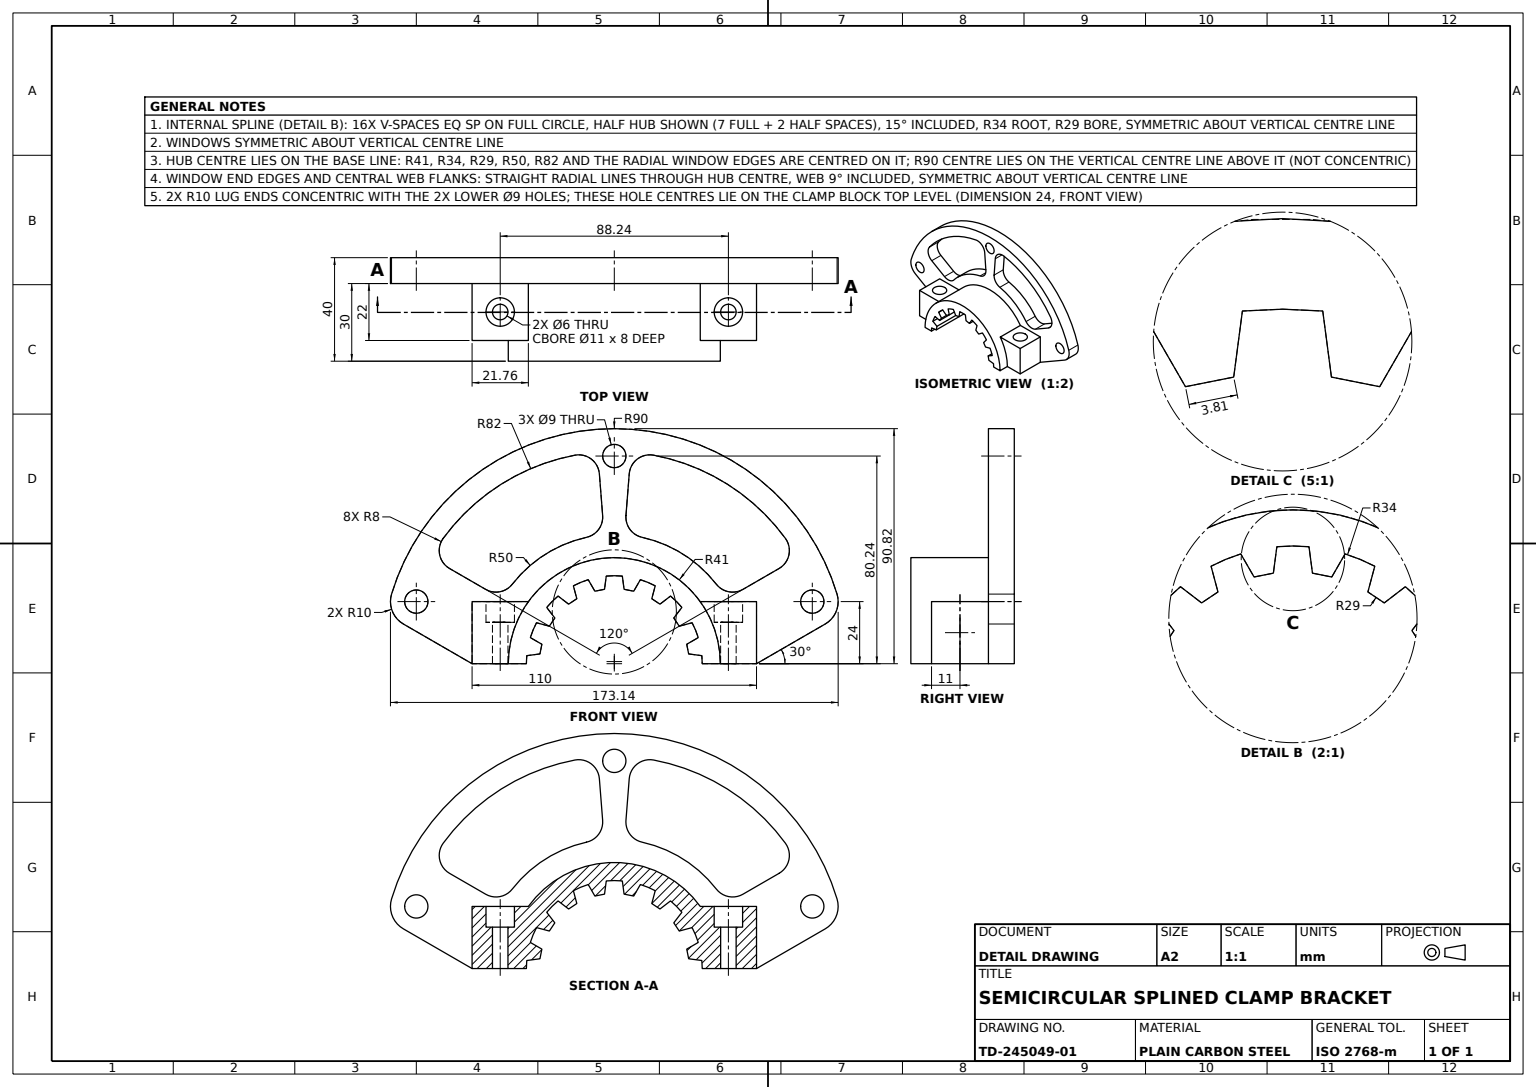
solid
v1 (-10.76075,48.828334,10)
v2 (-10.76075,48.828334,0)
e1 v1 v2 LINE
v3 (-39.439114,30.733635,0)
e2 v3 v2 CIRCLE(AX(P(0,0,0),D(0,0,-1),D(-1,0,0)),50)
v4 (-39.439114,30.733635,10)
e3 v4 v3 LINE
e4 v4 v1 CIRCLE(AX(P(0,0,10),D(0,0,-1),D(-1,0,0)),50)
face CYL(AX(P(0,0,10),D(0,0,-1),D(-1,0,0)),50) [e1 -e2 -e3 e4]
v5 (44.12077,16,26.5)
v6 (44.12077,24,26.5)
e5 v5 v6 LINE
v7 (44.12077,16,15.5)
e6 v7 v5 CIRCLE(AX(P(44.12077,16,21),D(0,1,0),D(0,0,1)),5.5)
v8 (44.12077,24,15.5)
e7 v7 v8 LINE
e8 v8 v6 CIRCLE(AX(P(44.12077,24,21),D(0,1,0),D(0,0,1)),5.5)
face CYL(AX(P(44.12077,24,21),D(0,1,0),D(0,0,1)),5.5) rev [-e5 -e6 e7 e8]
v9 (28.010307,7.511504,40)
v10 (28.752678,3.779355,40)
e9 v9 v10 CIRCLE(AX(P(0,0,40),D(0,0,-1),D(1,0,0)),29)
v11 (28.010307,7.511504,0)
e10 v11 v9 LINE
v12 (28.752678,3.779355,0)
e11 v11 v12 CIRCLE(AX(P(0,0,0),D(0,0,-1),D(1,0,0)),29)
e12 v12 v10 LINE
face CYL(AX(P(0,0,0),D(0,0,1),D(1,0,0)),29) rev [-e9 -e10 e11 e12]
v13 (-86.140372,26.897075,10)
v14 (-86.140372,26.897075,0)
e13 v13 v14 LINE
v15 (-86.569219,24,0)
e14 v14 v15 CIRCLE(AX(P(-76.569219,24,0),D(0,0,1),D(-1,0,0)),10)
v16 (-86.569219,24,10)
e15 v16 v15 LINE
e16 v13 v16 CIRCLE(AX(P(-76.569219,24,10),D(0,0,1),D(-1,0,0)),10)
face CYL(AX(P(-76.569219,24,10),D(0,0,-1),D(-1,0,0)),10) [e13 e14 -e15 -e16]
v17 (-33.24154,24,10)
v18 (-33.24154,24,32)
e17 v17 v18 LINE
v19 (-41,0,32)
e18 v18 v19 CIRCLE(AX(P(0,0,32),D(0,0,1),D(-1,0,0)),41)
v20 (-41,0,40)
e19 v20 v19 LINE
v21 (41,0,40)
e20 v21 v20 CIRCLE(AX(P(0,0,40),D(0,0,1),D(-1,0,0)),41)
v22 (41,0,32)
e21 v21 v22 LINE
v23 (33.24154,24,32)
e22 v22 v23 CIRCLE(AX(P(0,0,32),D(0,0,1),D(-1,0,0)),41)
v24 (33.24154,24,10)
e23 v23 v24 LINE
e24 v24 v17 CIRCLE(AX(P(0,0,10),D(0,0,1),D(-1,0,0)),41)
face CYL(AX(P(0,0,40),D(0,0,-1),D(-1,0,0)),41) [e17 e18 -e19 -e20 e21 e22 e23 e24]
v25 (-81.569219,15.339746,0)
e25 v15 v25 CIRCLE(AX(P(-76.569219,24,0),D(0,0,1),D(-1,0,0)),10)
v26 (-81.569219,15.339746,10)
e26 v26 v25 LINE
e27 v16 v26 CIRCLE(AX(P(-76.569219,24,10),D(0,0,1),D(-1,0,0)),10)
face CYL(AX(P(-76.569219,24,10),D(0,0,-1),D(-1,0,0)),10) [e15 e25 -e26 -e27]
v27 (32.469549,10.086049,0)
v28 (32.469549,10.086049,40)
e28 v27 v28 LINE
v29 (30.091352,15.827525,40)
e29 v29 v28 CIRCLE(AX(P(0,0,40),D(0,0,-1),D(1,0,0)),34)
v30 (30.091352,15.827525,0)
e30 v30 v29 LINE
e31 v30 v27 CIRCLE(AX(P(0,0,0),D(0,0,-1),D(1,0,0)),34)
face CYL(AX(P(0,0,0),D(0,0,1),D(1,0,0)),34) rev [e28 -e29 -e30 e31]
v31 (10.76075,48.828334,0)
v32 (39.439114,30.733635,0)
e32 v31 v32 CIRCLE(AX(P(0,0,0),D(0,0,-1),D(-1,0,0)),50)
v33 (10.76075,48.828334,10)
e33 v33 v31 LINE
v34 (39.439114,30.733635,10)
e34 v33 v34 CIRCLE(AX(P(0,0,10),D(0,0,-1),D(-1,0,0)),50)
e35 v34 v32 LINE
face CYL(AX(P(0,0,10),D(0,0,-1),D(-1,0,0)),50) [-e32 -e33 e34 e35]
v35 (-55,0,0)
e36 v25 v35 LINE
v36 (-55,0,10)
e37 v36 v35 LINE
e38 v26 v36 LINE
face PLANE(AX(P(-55,0,10),D(0.5,0.866025404,0),D(-0.866025404,0.5,0))) rev [e26 e36 -e37 -e38]
v37 (-25.117714,14.494842,0)
v38 (-25.117714,14.494842,40)
e39 v37 v38 LINE
v39 (-30.091352,15.827525,40)
e40 v39 v38 LINE
v40 (-30.091352,15.827525,0)
e41 v40 v39 LINE
e42 v40 v37 LINE
face PLANE(AX(P(1.941143,7.244444,0),D(-0.258819045,-0.965925826,0),D(0.965925826,-0.258819045,0))) [e39 -e40 -e41 e42]
v41 (3.107264,33.857716,40)
v42 (3.779355,28.752678,40)
e43 v41 v42 LINE
v43 (3.107264,33.857716,0)
e44 v43 v41 LINE
v44 (3.779355,28.752678,0)
e45 v43 v44 LINE
e46 v44 v42 LINE
face PLANE(AX(P(7.435836,0.978946,0),D(-0.991444861,-0.130526192,0),D(0.130526192,-0.991444861,0))) [-e43 -e44 e45 e46]
v45 (17.658806,23.003621,0)
v46 (17.658806,23.003621,40)
e47 v45 v46 LINE
v47 (14.494842,25.117714,40)
e48 v47 v46 CIRCLE(AX(P(0,0,40),D(0,0,-1),D(1,0,0)),29)
v48 (14.494842,25.117714,0)
e49 v48 v47 LINE
e50 v48 v45 CIRCLE(AX(P(0,0,0),D(0,0,-1),D(1,0,0)),29)
face CYL(AX(P(0,0,0),D(0,0,1),D(1,0,0)),29) rev [e47 -e48 -e49 e50]
v49 (-72.069219,24,10)
v50 (-72.069219,24,0)
e51 v49 v50 LINE
v51 (-81.069219,24,10)
e52 v49 v51 CIRCLE(AX(P(-76.569219,24,10),D(0,0,1),D(1,0,0)),4.5)
v52 (-81.069219,24,0)
e53 v51 v52 LINE
e54 v50 v52 CIRCLE(AX(P(-76.569219,24,0),D(0,0,1),D(1,0,0)),4.5)
face CYL(AX(P(-76.569219,24,10),D(0,0,-1),D(-1,0,0)),4.5) rev [-e51 e52 e53 -e54]
v53 (-23.003621,17.658806,40)
e55 v38 v53 CIRCLE(AX(P(0,0,40),D(0,0,-1),D(1,0,0)),29)
v54 (-23.003621,17.658806,0)
e56 v37 v54 CIRCLE(AX(P(0,0,0),D(0,0,-1),D(1,0,0)),29)
e57 v54 v53 LINE
face CYL(AX(P(0,0,0),D(0,0,1),D(1,0,0)),29) rev [-e55 -e39 e56 e57]
v55 (-4.5,80.242416,10)
v56 (4.5,80.242416,10)
e58 v55 v56 CIRCLE(AX(P(0,80.242416,10),D(0,0,1),D(1,0,0)),4.5)
v57 (4.5,80.242416,0)
e59 v56 v57 LINE
v58 (-4.5,80.242416,0)
e60 v58 v57 CIRCLE(AX(P(0,80.242416,0),D(0,0,1),D(1,0,0)),4.5)
e61 v55 v58 LINE
face CYL(AX(P(0,80.242416,10),D(0,0,-1),D(-1,0,0)),4.5) rev [e58 e59 -e60 -e61]
v59 (55,0,32)
v60 (55,0,10)
e62 v59 v60 LINE
e63 v22 v59 LINE
v61 (34,0,40)
e64 v61 v21 LINE
v62 (34,0,0)
e65 v62 v61 LINE
v63 (55,0,0)
e66 v62 v63 LINE
e67 v60 v63 LINE
v64 (44.12077,0,24)
v65 (44.12077,0,18)
e68 v64 v65 CIRCLE(AX(P(44.12077,0,21),D(0,1,0),D(-1,0,0)),3)
e69 v65 v64 CIRCLE(AX(P(44.12077,0,21),D(0,1,0),D(-1,0,0)),3)
face PLANE(AX(P(0,0,10),D(0,1,0),D(-1,0,0))) rev [-e62 -e63 -e21 -e64 -e65 e66 -e67] [e68 e69]
v66 (49.749372,28.722813,10)
e70 v34 v66 CIRCLE(AX(P(45.749372,35.651016,10),D(0,0,1),D(1,0,0)),8)
v67 (49.749372,28.722813,0)
e71 v66 v67 LINE
e72 v32 v67 CIRCLE(AX(P(45.749372,35.651016,0),D(0,0,1),D(1,0,0)),8)
face CYL(AX(P(45.749372,35.651016,10),D(0,0,-1),D(-1,0,0)),8) rev [-e35 e70 e71 -e72]
v68 (55,24,32)
e73 v59 v68 LINE
e74 v68 v23 LINE
face PLANE(AX(P(0,0,32),D(0,0,-1),D(-1,0,0))) rev [e73 e74 -e22 e63]
v69 (-26.138188,21.743853,0)
e75 v69 v54 LINE
v70 (-26.138188,21.743853,40)
e76 v69 v70 LINE
e77 v70 v53 LINE
face PLANE(AX(P(-5.95015,-4.565711,0),D(-0.79335334,-0.608761429,0),D(0.608761429,-0.79335334,0))) rev [-e57 -e75 e76 e77]
v71 (10.086049,32.469549,0)
v72 (15.827525,30.091352,0)
e78 v71 v72 CIRCLE(AX(P(0,0,0),D(0,0,-1),D(1,0,0)),34)
v73 (15.827525,30.091352,40)
e79 v72 v73 LINE
v74 (10.086049,32.469549,40)
e80 v74 v73 CIRCLE(AX(P(0,0,40),D(0,0,-1),D(1,0,0)),34)
e81 v71 v74 LINE
face CYL(AX(P(0,0,0),D(0,0,1),D(1,0,0)),34) rev [e78 e79 -e80 -e81]
v75 (72.069219,24,0)
v76 (81.069219,24,0)
e82 v75 v76 CIRCLE(AX(P(76.569219,24,0),D(0,0,1),D(1,0,0)),4.5)
e83 v76 v75 CIRCLE(AX(P(76.569219,24,0),D(0,0,1),D(1,0,0)),4.5)
e84 v72 v48 LINE
v77 (7.511504,28.010307,0)
e85 v71 v77 LINE
e86 v44 v77 CIRCLE(AX(P(0,0,0),D(0,0,-1),D(1,0,0)),29)
v78 (-3.107264,33.857716,0)
e87 v78 v43 CIRCLE(AX(P(0,0,0),D(0,0,-1),D(1,0,0)),34)
v79 (-3.779355,28.752678,0)
e88 v78 v79 LINE
v80 (-7.511504,28.010307,0)
e89 v80 v79 CIRCLE(AX(P(0,0,0),D(0,0,-1),D(1,0,0)),29)
v81 (-10.086049,32.469549,0)
e90 v81 v80 LINE
v82 (-15.827525,30.091352,0)
e91 v81 v82 CIRCLE(AX(P(0,0,0),D(0,0,1),D(1,0,0)),34)
v83 (-14.494842,25.117714,0)
e92 v82 v83 LINE
v84 (-17.658806,23.003621,0)
e93 v84 v83 CIRCLE(AX(P(0,0,0),D(0,0,-1),D(1,0,0)),29)
v85 (-21.743853,26.138188,0)
e94 v85 v84 LINE
e95 v85 v69 CIRCLE(AX(P(0,0,0),D(0,0,1),D(1,0,0)),34)
v86 (-32.469549,10.086049,0)
e96 v40 v86 CIRCLE(AX(P(0,0,0),D(0,0,1),D(1,0,0)),34)
v87 (-28.010307,7.511504,0)
e97 v86 v87 LINE
v88 (-28.752678,3.779355,0)
e98 v88 v87 CIRCLE(AX(P(0,0,0),D(0,0,-1),D(1,0,0)),29)
v89 (-33.857716,3.107264,0)
e99 v89 v88 LINE
v90 (-34,0,0)
e100 v89 v90 CIRCLE(AX(P(0,0,0),D(0,0,1),D(1,0,0)),34)
e101 v35 v90 LINE
v91 (86.140372,26.897075,0)
e102 v91 v14 CIRCLE(AX(P(0,0.823403,0),D(0,0,1),D(-1,0,0)),90)
v92 (81.569219,15.339746,0)
e103 v92 v91 CIRCLE(AX(P(76.569219,24,0),D(0,0,1),D(1,0,0)),10)
e104 v63 v92 LINE
v93 (33.857716,3.107264,0)
e105 v93 v62 CIRCLE(AX(P(0,0,0),D(0,0,-1),D(1,0,0)),34)
e106 v93 v12 LINE
e107 v27 v11 LINE
v94 (25.117714,14.494842,0)
e108 v30 v94 LINE
v95 (23.003621,17.658806,0)
e109 v95 v94 CIRCLE(AX(P(0,0,0),D(0,0,-1),D(1,0,0)),29)
v96 (26.138188,21.743853,0)
e110 v96 v95 LINE
v97 (21.743853,26.138188,0)
e111 v97 v96 CIRCLE(AX(P(0,0,0),D(0,0,-1),D(1,0,0)),34)
e112 v97 v45 LINE
v98 (-66.165447,48.436903,0)
v99 (-67.710282,43.711352,0)
e113 v98 v99 CIRCLE(AX(P(-59.710282,43.711352,0),D(0,0,1),D(1,0,0)),8)
v100 (-63.710282,36.783148,0)
e114 v99 v100 CIRCLE(AX(P(-59.710282,43.711352,0),D(0,0,1),D(1,0,0)),8)
v101 (-49.749372,28.722813,0)
e115 v100 v101 LINE
e116 v101 v3 CIRCLE(AX(P(-45.749372,35.651016,0),D(0,0,1),D(-1,0,0)),8)
v102 (-4.507132,57.268541,0)
e117 v2 v102 CIRCLE(AX(P(-12.482471,56.640868,0),D(0,0,1),D(-1,0,0)),8)
v103 (-5.771945,73.339516,0)
e118 v102 v103 LINE
v104 (-15.233477,80.572583,0)
e119 v103 v104 CIRCLE(AX(P(-13.747284,72.711844,0),D(0,0,1),D(1,0,0)),8)
e120 v104 v98 CIRCLE(AX(P(0,0,0),D(0,0,1),D(1,0,0)),82)
e121 v57 v58 CIRCLE(AX(P(0,80.242416,0),D(0,0,1),D(1,0,0)),4.5)
e122 v52 v50 CIRCLE(AX(P(-76.569219,24,0),D(0,0,1),D(1,0,0)),4.5)
v105 (63.710282,36.783148,0)
e123 v67 v105 LINE
v106 (66.165447,48.436903,0)
e124 v105 v106 CIRCLE(AX(P(59.710282,43.711352,0),D(0,0,1),D(1,0,0)),8)
v107 (15.233477,80.572583,0)
e125 v106 v107 CIRCLE(AX(P(0,0,0),D(0,0,1),D(1,0,0)),82)
v108 (5.771945,73.339516,0)
e126 v107 v108 CIRCLE(AX(P(13.747284,72.711844,0),D(0,0,1),D(-1,0,0)),8)
v109 (4.507132,57.268541,0)
e127 v108 v109 LINE
v110 (4.482471,56.640868,0)
e128 v109 v110 CIRCLE(AX(P(12.482471,56.640868,0),D(0,0,1),D(1,0,0)),8)
e129 v110 v31 CIRCLE(AX(P(12.482471,56.640868,0),D(0,0,1),D(1,0,0)),8)
face PLANE(AX(P(-76.569219,24,0),D(0,0,-1),D(-1,0,0))) [e82 e83] [-e50 -e84 -e78 e85 -e86 -e45 -e87 e88 -e89 -e90 e91 e92 -e93 -e94 e95 e75 -e56 -e42 e96 e97 -e98 -e99 e100 -e101 -e36 -e25 -e14 -e102 -e103 -e104 -e66 -e105 e106 -e11 -e107 -e31 e108 -e109 -e110 -e111 e112] [e113 e114 e115 e116 e2 e117 e118 e119 e120] [e60 e121] [e54 e122] [e123 e124 e125 e126 e127 e128 e129 e32 e72]
v111 (-3.779355,28.752678,40)
e130 v79 v111 LINE
v112 (-7.511504,28.010307,40)
e131 v112 v111 CIRCLE(AX(P(0,0,40),D(0,0,-1),D(1,0,0)),29)
e132 v80 v112 LINE
face CYL(AX(P(0,0,0),D(0,0,1),D(1,0,0)),29) rev [e89 e130 -e131 -e132]
v113 (25.117714,14.494842,40)
e133 v29 v113 LINE
e134 v94 v113 LINE
face PLANE(AX(P(-1.941143,7.244444,0),D(-0.258819045,0.965925826,0),D(-0.965925826,-0.258819045,0))) rev [-e108 e30 e133 -e134]
v114 (44.12077,16,24)
e135 v64 v114 LINE
v115 (44.12077,16,18)
e136 v114 v115 CIRCLE(AX(P(44.12077,16,21),D(0,1,0),D(0,0,1)),3)
e137 v65 v115 LINE
face CYL(AX(P(44.12077,24,21),D(0,1,0),D(0,0,1)),3) rev [e135 e136 -e137 -e68]
v116 (33.857716,3.107264,40)
e138 v93 v116 LINE
e139 v116 v10 LINE
face PLANE(AX(P(0.978946,7.435836,0),D(0.130526192,0.991444861,0),D(-0.991444861,0.130526192,0))) rev [e138 e139 -e12 -e106]
v117 (-28.010307,7.511504,40)
e140 v87 v117 LINE
v118 (-32.469549,10.086049,40)
e141 v86 v118 LINE
e142 v118 v117 LINE
face PLANE(AX(P(-3.75,-6.495191,0),D(-0.5,-0.866025404,0),D(0.866025404,-0.5,0))) rev [-e140 -e97 e141 e142]
v119 (-14.494842,25.117714,40)
e143 v83 v119 LINE
v120 (-17.658806,23.003621,40)
e144 v120 v119 CIRCLE(AX(P(0,0,40),D(0,0,-1),D(1,0,0)),29)
e145 v84 v120 LINE
face CYL(AX(P(0,0,0),D(0,0,1),D(1,0,0)),29) rev [e143 -e144 -e145 e93]
v121 (-3.107264,33.857716,40)
e146 v78 v121 LINE
e147 v121 v111 LINE
face PLANE(AX(P(-7.435836,0.978946,0),D(-0.991444861,0.130526192,0),D(-0.130526192,-0.991444861,0))) rev [-e130 -e88 e146 e147]
v122 (81.569219,15.339746,10)
v123 (86.140372,26.897075,10)
e148 v122 v123 CIRCLE(AX(P(76.569219,24,10),D(0,0,1),D(1,0,0)),10)
e149 v122 v92 LINE
e150 v123 v91 LINE
face CYL(AX(P(76.569219,24,10),D(0,0,-1),D(-1,0,0)),10) [-e148 e149 e103 -e150]
v124 (-63.710282,36.783148,10)
e151 v124 v100 LINE
v125 (-49.749372,28.722813,10)
e152 v124 v125 LINE
e153 v125 v101 LINE
face PLANE(AX(P(-49.749372,28.722813,10),D(0.5,0.866025404,0),D(-0.866025404,0.5,0))) [-e151 e152 e153 -e115]
v126 (-4.507132,57.268541,10)
e154 v126 v102 LINE
v127 (-5.771945,73.339516,10)
e155 v126 v127 LINE
e156 v127 v103 LINE
face PLANE(AX(P(-4.507132,57.268541,10),D(-0.996917334,-0.078459096,0),D(0.078459096,-0.996917334,0))) [-e118 -e154 e155 e156]
v128 (-21.743853,26.138188,40)
e157 v128 v70 CIRCLE(AX(P(0,0,40),D(0,0,1),D(1,0,0)),34)
e158 v85 v128 LINE
face CYL(AX(P(0,0,0),D(0,0,1),D(1,0,0)),34) rev [e157 -e76 -e95 e158]
v129 (-44.12077,24,26.5)
v130 (-44.12077,24,15.5)
e159 v129 v130 CIRCLE(AX(P(-44.12077,24,21),D(0,1,0),D(0,0,1)),5.5)
v131 (-44.12077,16,15.5)
e160 v131 v130 LINE
v132 (-44.12077,16,26.5)
e161 v132 v131 CIRCLE(AX(P(-44.12077,16,21),D(0,1,0),D(0,0,1)),5.5)
e162 v132 v129 LINE
face CYL(AX(P(-44.12077,24,21),D(0,1,0),D(0,0,1)),5.5) rev [e159 -e160 -e161 e162]
v133 (-15.827525,30.091352,40)
e163 v82 v133 LINE
v134 (-10.086049,32.469549,40)
e164 v81 v134 LINE
e165 v134 v133 CIRCLE(AX(P(0,0,40),D(0,0,1),D(1,0,0)),34)
face CYL(AX(P(0,0,0),D(0,0,1),D(1,0,0)),34) rev [-e163 -e91 e164 e165]
e166 v6 v8 CIRCLE(AX(P(44.12077,24,21),D(0,1,0),D(0,0,1)),5.5)
e167 v5 v7 CIRCLE(AX(P(44.12077,16,21),D(0,1,0),D(0,0,1)),5.5)
face CYL(AX(P(44.12077,24,21),D(0,1,0),D(0,0,1)),5.5) rev [e5 e166 -e7 -e167]
e168 v130 v129 CIRCLE(AX(P(-44.12077,24,21),D(0,1,0),D(0,0,1)),5.5)
e169 v131 v132 CIRCLE(AX(P(-44.12077,16,21),D(0,1,0),D(0,0,1)),5.5)
face CYL(AX(P(-44.12077,24,21),D(0,1,0),D(0,0,1)),5.5) rev [e168 -e162 -e169 e160]
e170 v60 v122 LINE
face PLANE(AX(P(55,0,10),D(-0.5,0.866025404,0),D(-0.866025404,-0.5,0))) rev [-e170 e67 e104 -e149]
e171 v39 v118 CIRCLE(AX(P(0,0,40),D(0,0,1),D(1,0,0)),34)
face CYL(AX(P(0,0,0),D(0,0,1),D(1,0,0)),34) rev [-e141 -e96 e41 e171]
v135 (55,24,10)
e172 v135 v24 LINE
e173 v68 v135 LINE
face PLANE(AX(P(-55,24,32),D(0,-1,0),D(0,0,-1))) rev [e172 -e23 -e74 e173] [-e8 -e166]
e174 v125 v4 CIRCLE(AX(P(-45.749372,35.651016,10),D(0,0,1),D(-1,0,0)),8)
face CYL(AX(P(-45.749372,35.651016,10),D(0,0,-1),D(-1,0,0)),8) rev [-e116 -e153 e174 e3]
e175 v121 v41 CIRCLE(AX(P(0,0,40),D(0,0,-1),D(1,0,0)),34)
face CYL(AX(P(0,0,0),D(0,0,1),D(1,0,0)),34) rev [-e175 -e146 e87 e44]
v136 (63.710282,36.783148,10)
e176 v136 v105 LINE
e177 v66 v136 LINE
face PLANE(AX(P(49.749372,28.722813,10),D(-0.5,0.866025404,0),D(-0.866025404,-0.5,0))) [e176 -e123 -e71 e177]
v137 (-67.710282,43.711352,10)
e178 v137 v99 LINE
e179 v137 v124 CIRCLE(AX(P(-59.710282,43.711352,10),D(0,0,1),D(1,0,0)),8)
face CYL(AX(P(-59.710282,43.711352,10),D(0,0,-1),D(-1,0,0)),8) rev [-e114 -e178 e179 e151]
v138 (-44.12077,16,18)
v139 (-44.12077,16,24)
e180 v138 v139 CIRCLE(AX(P(-44.12077,16,21),D(0,1,0),D(0,0,1)),3)
e181 v139 v138 CIRCLE(AX(P(-44.12077,16,21),D(0,1,0),D(0,0,1)),3)
face PLANE(AX(P(-41.12077,16,21),D(0,-1,0),D(0,0,-1))) rev [e161 e169] [-e180 -e181]
v140 (72.069219,24,10)
e182 v140 v75 LINE
v141 (81.069219,24,10)
e183 v140 v141 CIRCLE(AX(P(76.569219,24,10),D(0,0,1),D(1,0,0)),4.5)
e184 v141 v76 LINE
face CYL(AX(P(76.569219,24,10),D(0,0,-1),D(-1,0,0)),4.5) rev [-e82 -e182 e183 e184]
v142 (-15.233477,80.572583,10)
e185 v127 v142 CIRCLE(AX(P(-13.747284,72.711844,10),D(0,0,1),D(1,0,0)),8)
e186 v142 v104 LINE
face CYL(AX(P(-13.747284,72.711844,10),D(0,0,-1),D(-1,0,0)),8) rev [-e156 e185 e186 -e119]
e187 v115 v114 CIRCLE(AX(P(44.12077,16,21),D(0,1,0),D(0,0,1)),3)
face PLANE(AX(P(47.12077,16,21),D(0,-1,0),D(0,0,-1))) rev [e167 e6] [-e136 -e187]
e188 v116 v61 CIRCLE(AX(P(0,0,40),D(0,0,-1),D(1,0,0)),34)
face CYL(AX(P(0,0,0),D(0,0,1),D(1,0,0)),34) rev [-e188 -e138 e105 e65]
v143 (-55,24,32)
v144 (-55,24,10)
e189 v143 v144 LINE
e190 v18 v143 LINE
e191 v17 v144 LINE
face PLANE(AX(P(-55,24,32),D(0,-1,0),D(0,0,-1))) rev [-e159 -e168] [-e189 -e190 -e17 e191]
v145 (7.511504,28.010307,40)
e192 v74 v145 LINE
e193 v77 v145 LINE
face PLANE(AX(P(-6.495191,3.75,0),D(-0.866025404,0.5,0),D(-0.5,-0.866025404,0))) rev [e192 -e193 -e85 e81]
v146 (15.233477,80.572583,10)
e194 v146 v107 LINE
v147 (5.771945,73.339516,10)
e195 v146 v147 CIRCLE(AX(P(13.747284,72.711844,10),D(0,0,1),D(-1,0,0)),8)
e196 v147 v108 LINE
face CYL(AX(P(13.747284,72.711844,10),D(0,0,-1),D(-1,0,0)),8) rev [-e126 -e194 e195 e196]
v148 (-34,0,40)
e197 v20 v148 LINE
v149 (-33.857716,3.107264,40)
e198 v149 v148 CIRCLE(AX(P(0,0,40),D(0,0,1),D(1,0,0)),34)
v150 (-28.752678,3.779355,40)
e199 v149 v150 LINE
e200 v150 v117 CIRCLE(AX(P(0,0,40),D(0,0,-1),D(1,0,0)),29)
e201 v128 v120 LINE
e202 v133 v119 LINE
e203 v134 v112 LINE
e204 v42 v145 CIRCLE(AX(P(0,0,40),D(0,0,-1),D(1,0,0)),29)
e205 v73 v47 LINE
v151 (21.743853,26.138188,40)
e206 v151 v46 LINE
v152 (26.138188,21.743853,40)
e207 v151 v152 CIRCLE(AX(P(0,0,40),D(0,0,-1),D(1,0,0)),34)
v153 (23.003621,17.658806,40)
e208 v152 v153 LINE
e209 v153 v113 CIRCLE(AX(P(0,0,40),D(0,0,-1),D(1,0,0)),29)
e210 v28 v9 LINE
face PLANE(AX(P(0,0,40),D(0,0,-1),D(-1,0,0))) rev [e20 e197 -e198 e199 e200 -e142 -e171 e40 e55 -e77 -e157 e201 e144 -e202 -e165 e203 e131 -e147 e175 e43 e204 -e192 e80 e205 e48 -e206 e207 e208 e209 -e133 e29 e210 e9 -e139 e188 e64]
v154 (-44.12077,0,24)
v155 (-44.12077,0,18)
e211 v154 v155 CIRCLE(AX(P(-44.12077,0,21),D(0,1,0),D(-1,0,0)),3)
e212 v154 v139 LINE
e213 v155 v138 LINE
face CYL(AX(P(-44.12077,24,21),D(0,1,0),D(0,0,1)),3) rev [-e211 e212 e181 -e213]
v156 (-66.165447,48.436903,10)
e214 v156 v98 LINE
e215 v156 v137 CIRCLE(AX(P(-59.710282,43.711352,10),D(0,0,1),D(1,0,0)),8)
face CYL(AX(P(-59.710282,43.711352,10),D(0,0,-1),D(-1,0,0)),8) rev [e178 -e113 -e214 e215]
e216 v60 v135 LINE
e217 v123 v13 CIRCLE(AX(P(0,0.823403,10),D(0,0,1),D(-1,0,0)),90)
e218 v144 v36 LINE
e219 v141 v140 CIRCLE(AX(P(76.569219,24,10),D(0,0,1),D(1,0,0)),4.5)
e220 v142 v156 CIRCLE(AX(P(0,0,10),D(0,0,1),D(1,0,0)),82)
e221 v1 v126 CIRCLE(AX(P(-12.482471,56.640868,10),D(0,0,1),D(-1,0,0)),8)
e222 v56 v55 CIRCLE(AX(P(0,80.242416,10),D(0,0,1),D(1,0,0)),4.5)
e223 v51 v49 CIRCLE(AX(P(-76.569219,24,10),D(0,0,1),D(1,0,0)),4.5)
v157 (4.507132,57.268541,10)
e224 v147 v157 LINE
v158 (66.165447,48.436903,10)
e225 v158 v146 CIRCLE(AX(P(0,0,10),D(0,0,1),D(1,0,0)),82)
e226 v136 v158 CIRCLE(AX(P(59.710282,43.711352,10),D(0,0,1),D(1,0,0)),8)
v159 (4.482471,56.640868,10)
e227 v159 v33 CIRCLE(AX(P(12.482471,56.640868,10),D(0,0,1),D(1,0,0)),8)
e228 v157 v159 CIRCLE(AX(P(12.482471,56.640868,10),D(0,0,1),D(1,0,0)),8)
face PLANE(AX(P(-76.569219,24,10),D(0,0,-1),D(-1,0,0))) rev [-e172 -e216 e170 e148 e217 e16 e27 e38 -e218 -e191 -e24] [-e219 -e183] [-e174 -e152 -e179 -e215 -e220 -e185 -e155 -e221 -e4] [-e58 -e222] [-e223 -e52] [-e224 -e195 -e225 -e226 -e177 -e70 -e34 -e227 -e228]
e229 v159 v110 LINE
face CYL(AX(P(12.482471,56.640868,10),D(0,0,-1),D(-1,0,0)),8) rev [e33 -e129 -e229 e227]
e230 v157 v109 LINE
face PLANE(AX(P(4.507132,57.268541,10),D(0.996917334,-0.078459096,0),D(0.078459096,0.996917334,0))) [e230 -e127 -e196 e224]
e231 v88 v150 LINE
face CYL(AX(P(0,0,0),D(0,0,1),D(1,0,0)),29) rev [e140 -e200 -e231 e98]
e232 v158 v106 LINE
face CYL(AX(P(0,0,10),D(0,0,-1),D(-1,0,0)),82) rev [-e125 -e232 e225 e194]
face PLANE(AX(P(6.495191,3.75,0),D(-0.866025404,-0.5,0),D(0.5,-0.866025404,0))) [e132 -e203 -e164 e90]
face CYL(AX(P(0,0,0),D(0,0,1),D(1,0,0)),29) rev [e193 -e204 -e46 e86]
face PLANE(AX(P(4.565711,5.95015,0),D(-0.608761429,-0.79335334,0),D(0.79335334,-0.608761429,0))) [-e158 e94 e145 -e201]
face CYL(AX(P(76.569219,24,10),D(0,0,-1),D(-1,0,0)),4.5) rev [e219 e182 -e83 -e184]
face CYL(AX(P(44.12077,24,21),D(0,1,0),D(0,0,1)),3) rev [e137 e187 -e135 -e69]
face CYL(AX(P(-76.569219,24,10),D(0,0,-1),D(-1,0,0)),4.5) rev [-e53 e223 e51 -e122]
v160 (-55,0,32)
e233 v143 v160 LINE
e234 v160 v36 LINE
face PLANE(AX(P(-55,0,32),D(1,0,0),D(0,0,-1))) rev [-e233 e189 e218 -e234]
face CYL(AX(P(59.710282,43.711352,10),D(0,0,-1),D(-1,0,0)),8) rev [-e176 e226 e232 -e124]
e235 v90 v148 LINE
e236 v89 v149 LINE
face CYL(AX(P(0,0,0),D(0,0,1),D(1,0,0)),34) rev [-e235 -e100 e236 e198]
face PLANE(AX(P(55,0,32),D(-1,0,0),D(0,0,1))) rev [e62 e216 -e173 -e73]
e237 v97 v151 LINE
face PLANE(AX(P(-4.565711,5.95015,0),D(-0.608761429,0.79335334,0),D(-0.79335334,-0.608761429,0))) rev [-e112 e237 e206 -e47]
face PLANE(AX(P(-7.244444,-1.941143,0),D(-0.965925826,-0.258819045,0),D(0.258819045,-0.965925826,0))) rev [e202 -e143 -e92 e163]
face CYL(AX(P(0,0.823403,10),D(0,0,-1),D(-1,0,0)),90) [e150 e102 -e13 -e217]
face CYL(AX(P(12.482471,56.640868,10),D(0,0,-1),D(-1,0,0)),8) rev [e228 e229 -e128 -e230]
face PLANE(AX(P(3.75,-6.495191,0),D(-0.5,0.866025404,0),D(-0.866025404,-0.5,0))) [e107 e10 -e210 -e28]
face PLANE(AX(P(-0.978946,7.435836,0),D(0.130526192,-0.991444861,0),D(0.991444861,0.130526192,0))) [-e199 -e236 e99 e231]
e238 v155 v154 CIRCLE(AX(P(-44.12077,0,21),D(0,1,0),D(-1,0,0)),3)
face CYL(AX(P(-44.12077,24,21),D(0,1,0),D(0,0,1)),3) rev [e213 e180 -e212 -e238]
face CYL(AX(P(-12.482471,56.640868,10),D(0,0,-1),D(-1,0,0)),8) rev [-e117 -e1 e221 e154]
face CYL(AX(P(0,0,10),D(0,0,-1),D(-1,0,0)),82) rev [-e120 -e186 e220 e214]
e239 v160 v19 LINE
face PLANE(AX(P(0,0,10),D(0,1,0),D(-1,0,0))) rev [-e239 e234 e37 e101 e235 -e197 e19] [e238 e211]
face PLANE(AX(P(7.244444,-1.941143,0),D(-0.965925826,0.258819045,0),D(-0.258819045,-0.965925826,0))) [e84 e49 -e205 -e79]
e240 v96 v152 LINE
face CYL(AX(P(0,0,0),D(0,0,1),D(1,0,0)),34) rev [e240 -e207 -e237 e111]
e241 v95 v153 LINE
face CYL(AX(P(0,0,0),D(0,0,1),D(1,0,0)),29) rev [e109 e134 -e209 -e241]
face PLANE(AX(P(5.95015,-4.565711,0),D(-0.79335334,0.608761429,0),D(-0.608761429,-0.79335334,0))) [-e208 -e240 e110 e241]
face CYL(AX(P(0,80.242416,10),D(0,0,-1),D(-1,0,0)),4.5) rev [e222 e61 -e121 -e59]
face PLANE(AX(P(0,0,32),D(0,0,-1),D(-1,0,0))) rev [e190 e233 e239 -e18]
